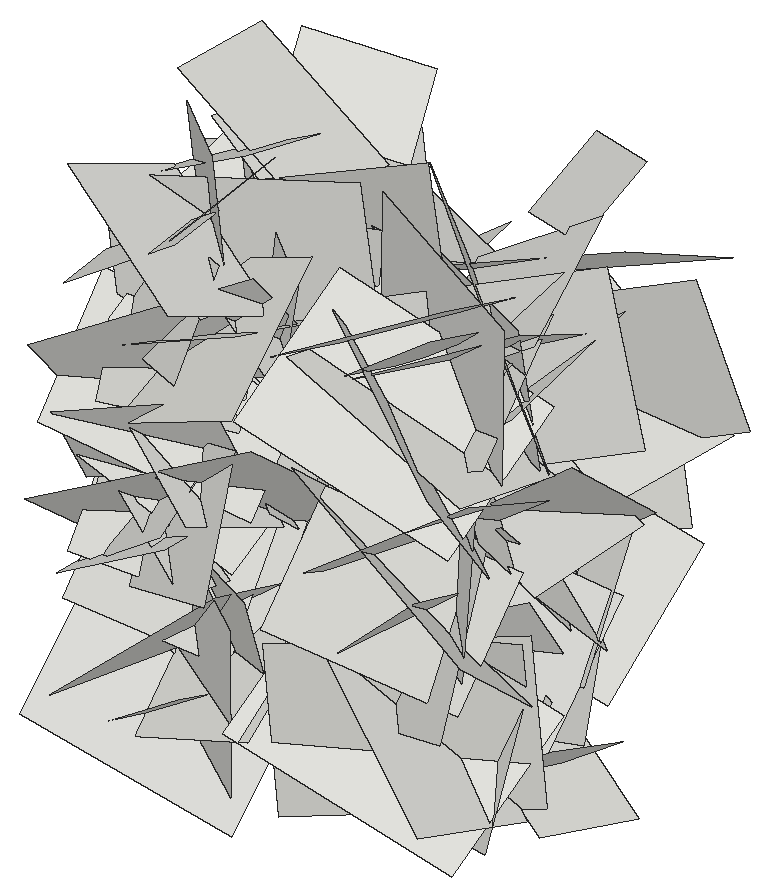
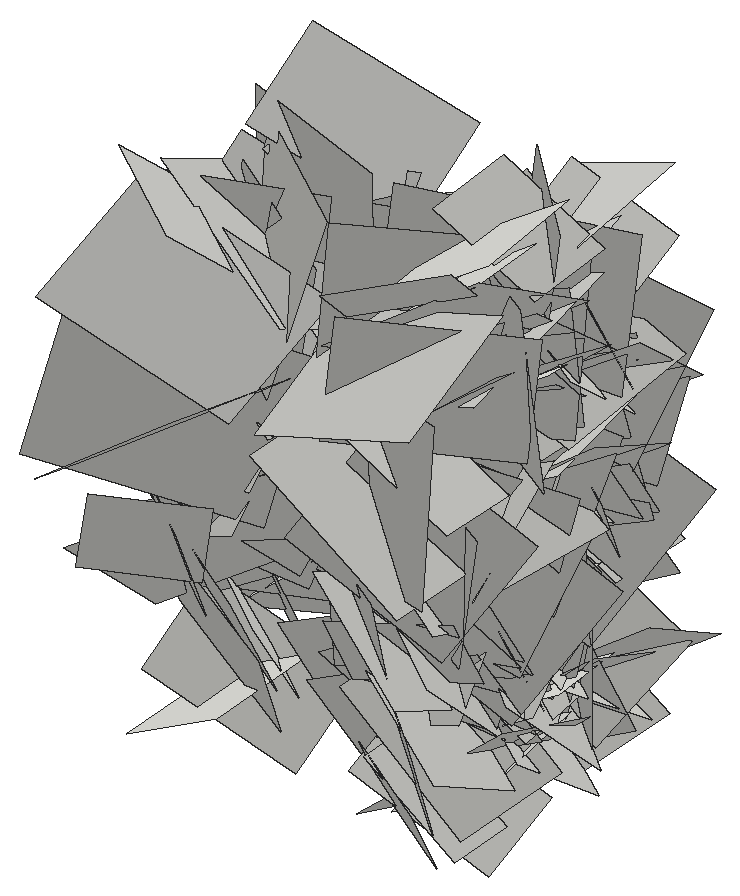
# SketchUp Ruby script. Lengths in inches.
U = 1.inch
M = Sketchup.active_model
def pt(a) = Geom::Point3d.new(a.map { |v| v * U })
def face(e, loops, mat)
  f = e.add_face(loops[0].map { |a| pt(a) })
  loops[1..].each { |l| e.add_face(l.map { |a| pt(a) }).erase! }
  f.material = f.back_material = mat if mat
  f
end
# faces: each face lists its corners as indices into pts; further lists are holes
def faces(e, pts, list, mat = nil) = list.each { |f| face(e, (f[0].is_a?(Array) ? f : [f]).map { |l| l.map { |i| pts[i] } }, mat) }
# xy, xz, yz: faces in a plane at the given z, y or x. An outline is a flat list of corners, or four numbers for a rectangle; further outlines are holes
def ring(l) = l.size == 4 ? [[l[0], l[1]], [l[2], l[1]], [l[2], l[3]], [l[0], l[3]]] : l.each_slice(2).to_a
def flat(e, list, mat, &to3) = list.each { |f| face(e, (f[0].is_a?(Array) ? f : [f]).map { |l| ring(l).map { |u, v| to3.(u, v) } }, mat) }
def xy(e, z, list, mat = nil) = flat(e, list, mat) { |x, y| [x, y, z] }
def xz(e, y, list, mat = nil) = flat(e, list, mat) { |x, z| [x, y, z] }
def yz(e, x, list, mat = nil) = flat(e, list, mat) { |y, z| [x, y, z] }
def lines(e, pts, list) = list.each { |a, b| e.add_line(pt(pts[a]), pt(pts[b])) }
# prism: a flat outline (further loops are holes) pulled along v
def prism(e, loops, v, mat = nil)
  f = face(e, loops, mat); d = Geom::Vector3d.new(v.map { |x| x * U })
  f.pushpull(f.normal.samedirection?(d) ? d.length : -d.length)
end
def box(e, o, s, mat = nil) = prism(e, [[o, [o[0] + s[0], o[1], o[2]], [o[0] + s[0], o[1] + s[1], o[2]], [o[0], o[1] + s[1], o[2]]]], [0, 0, s[2]], mat)
def at(x, y, z, deg = 0) = Geom::Transformation.translation(pt([x, y, z])) * Geom::Transformation.rotation(ORIGIN, Z_AXIS, deg.degrees)
def axes(o, x, y, z) = Geom::Transformation.new([*x, 0, *y, 0, *z, 0, *pt(o).to_a, 1])
def part(name) = M.definitions.add(name)
# library, detail: a bought-in or finely detailed component or shape, given as its bounding box
def library(name, o, s) = part(name).tap { |d| box(d.entities, o, s) }
def detail(e, o, s) = box(e.add_group.entities, o, s)
def put(e, d, t, mat = nil) = e.add_instance(d, t).tap { |i| i.material = mat if mat }
def group(e, t, mat = nil) = e.add_group.tap { |g| g.transformation = t; g.material = mat if mat }.entities
root = M.entities
c1 = part("Component\#6")
p = [[0.01,0,0],[0,3.24,4.54],[4.32,3.24,4.54],[4.33,0,0]]
faces(c1.entities,p,[[0,1,2,3]])
put(root,c1,axes([410.71,139.47,36.72],[0.15825,-0.66033,0.08813],[0.02764,0.09604,0.67542],[0.70562,0.14433,-0.04622]))
put(root,c1,axes([414.68,137.53,34.5],[0.08019,0.3809,0.76753],[-0.04804,0.77121,-0.37826],[-0.90698,-0.00717,0.08789]))
put(root,c1,axes([414.68,137.14,29.31],[-0.00249,0.75761,-0.01469],[-0.08098,-0.01485,-0.75375],[-0.79913,-0.00085,0.07643]))
put(root,c1,axes([414.68,149.44,28.46],[0.01637,-0.35652,-0.61871],[-0.18604,-0.60176,0.34238],[-0.7337,0.14463,-0.10062]))
put(root,c1,axes([410.71,144.76,23.61],[0.10873,-0.7568,0.02149],[-0.01122,0.02025,0.76368],[0.80245,0.10283,0.00777]))
put(root,c1,axes([414.68,139.84,37.375],[-0.13047,0.02824,0.77],[0.11824,0.77221,-0.01049],[-0.80815,0.10842,-0.12584]))
put(root,c1,axes([410.71,147.86,21.63],[-0.08807,-1.00346,0.13322],[-0.11481,0.14172,0.99989],[1.06685,-0.06759,0.1186]))
put(root,c1,axes([410.71,145.6875,25.3],[-0.21495,-0.77208,-0.77151],[-0.06755,-0.77499,0.79232],[1.15499,-0.18901,-0.09724]))
put(root,c1,axes([410.71,141.61,27.46],[-0.15544,0.8369,-0.58263],[-0.03072,-0.5918,-0.84279],[1.08048,0.10358,-0.10778]))
put(root,c1,axes([414.68,146.7,34.04],[0.22474,0.77203,-0.6543],[0.03576,-0.67353,-0.78378],[-1.07212,0.13937,-0.1633]))
put(root,c1,axes([414.68,140.76,35.5625],[-0.0095,0.80566,-0.00603],[0.04784,-0.00552,-0.80445],[-0.85268,-0.00929,-0.04507]))
put(root,c1,axes([414.68,144.98,23.12],[-0.11015,0.70988,0.06167],[0.04855,0.06885,-0.71532],[-0.75374,-0.09931,-0.05509]))
put(root,c1,axes([410.71,147.08,31.53],[-0.0186,0.21399,-0.90436],[-0.04027,-0.90393,-0.21315],[0.98427,-0.03294,-0.02581]))
put(root,c1,axes([410.71,137.85,30.84],[-0.06669,0.91948,0.38333],[-0.06841,0.37952,-0.92095],[1.05374,0.08283,-0.03553]))
put(root,c1,axes([414.68,143.64,28.51],[-0.01569,-0.00258,-0.72773],[-0.02057,-0.72762,0.00297],[-0.77112,0.01947,0.01473]))
put(root,c1,axes([410.71,144.71,33.13],[-0.16995,0.04512,1.05289],[-0.00982,1.0649,-0.04705],[1.11704,0.01623,0.15977]))
put(root,c1,axes([410.71,149.13,24.11],[-0.03147,-0.85153,-0.39996],[-0.02133,-0.3995,0.85202],[0.997,-0.03542,0.00561]))
put(root,c1,axes([410.71,150.98,27.43],[0.11329,-0.77541,-0.3635],[-0.07754,-0.37325,0.77469],[0.90445,0.06513,0.11195]))
put(root,c1,axes([410.71,138.53,29.67],[0.03677,-0.4198,0.69058],[0.10131,0.68849,0.41374],[0.85065,-0.06385,-0.07912]))
put(root,c1,axes([414.68,144.05,31.85],[0.11078,0.17753,-0.74918],[-0.12323,-0.74375,-0.19246],[-0.80677,0.13798,-0.07348]))
put(root,c1,axes([414.68,143.38,25.93],[0.00088,-0.66729,0.07011],[-0.1194,0.06898,0.65784],[-0.70113,-0.01259,-0.11194]))
put(root,c1,axes([414.68,140.84,40.56],[0.05261,0.712,-0.12967],[-0.10362,-0.12219,-0.70833],[-0.7601,0.06594,0.08758]))
put(root,c1,axes([410.71,148.52,32.35],[0.08011,-0.79067,-0.06214],[0.07476,-0.05548,0.79163],[0.83736,0.0806,-0.06473]))
put(root,c1,axes([410.71,142.67,41.25],[-0.05619,0.9574,-0.08237],[0.00834,-0.08206,-0.95886],[1.01856,0.05349,0.00331]))
put(root,c1,axes([414.68,144.6,22.65],[0.17478,-0.82558,-0.09028],[-0.09417,-0.10904,0.83495],[-0.87528,-0.15312,-0.10786]))
put(root,c1,axes([410.71,145.42,24.52],[-0.2647,-0.88765,0.75819],[-0.01358,0.77738,0.90589],[1.23735,-0.18136,0.17214]))
put(root,c1,axes([410.71,141.63,23.18],[-0.01995,1.00092,0.30572],[-0.13829,0.30114,-0.99396],[1.10071,0.05598,-0.11933]))
put(root,c1,axes([414.68,145.6,27.28],[-0.00806,0.29423,-0.56577],[-0.12293,-0.55701,-0.28812],[-0.6647,0.09945,0.06014]))
put(root,c1,axes([410.71,135.48,23.28],[-0.21581,1.04519,0.5846],[-0.09636,0.57779,-1.06467],[1.26577,0.22219,0.01862]))
put(root,c1,axes([414.68,143.53,22.21],[0.15224,-0.84766,-0.36991],[0.10957,-0.35729,0.85887],[-0.97421,-0.17265,0.03879]))
put(root,c1,axes([414.68,137.77,24.11],[0.1419,0.78136,-0.16109],[-0.04598,-0.15597,-0.79258],[-0.84441,0.13979,0.01609]))
put(root,c1,axes([410.71,136.3,32.46],[-0.17238,0.91042,0.71253],[-0.07022,0.71102,-0.92361],[1.22345,0.16908,0.04738]))
put(root,c1,axes([410.71,137.68,27.62],[0.00267,0.49736,0.77514],[0.05686,0.77375,-0.49665],[0.97459,-0.04651,0.02685]))
put(root,c1,axes([410.71,145.12,23.07],[-0.0526,-0.82286,-0.58821],[0.0059,-0.58914,0.82367],[1.07215,-0.03713,-0.03339]))
put(root,c1,axes([414.68,145.7,22.51],[0.08358,0.19729,0.79599],[0.0899,0.79341,-0.20506],[-0.86462,0.10156,0.05562]))
put(root,c1,axes([414.68,146.3,23.53],[0.0913,-0.50535,0.50896],[-0.05568,0.5068,0.51209],[-0.75823,-0.09807,0.02368]))
put(root,c1,axes([414.68,145.72,37.21],[-0.0202,-0.65006,0.07365],[0.02062,0.07308,0.65011],[-0.69316,0.02112,0.01719]))
put(root,c1,axes([414.68,141.16,33.73],[-0.01034,-0.20439,-0.70125],[0.11317,-0.69418,0.20085],[-0.76594,-0.09981,0.03914]))
put(root,c1,axes([410.71,149.17,29.19],[0.22051,-0.77582,-0.34275],[-0.07369,-0.36732,0.78924],[0.89602,0.16072,0.14925]))
put(root,c1,axes([414.68,144.18,33.46],[0.08879,-0.56105,-0.39599],[-0.0694,-0.40364,0.55803],[-0.72461,-0.03009,-0.10197]))
put(root,c1,axes([414.68,136.92,29.78],[-0.03864,0.57092,0.32429],[0.05823,0.3263,-0.56829],[-0.69355,-0.00442,-0.06578]))
put(root,c1,axes([414.68,146.45,21.25],[0.00375,0.2874,0.54008],[-0.0654,0.5375,-0.28562],[-0.64519,-0.05282,0.03209]))
put(root,c1,axes([414.68,144.73,33.27],[0.16555,-0.76551,-0.15352],[-0.02389,-0.16091,0.77946],[-0.82725,-0.14855,-0.05323]))
put(root,c1,axes([410.71,144.65,25.96],[0.15377,0.53431,0.65108],[0.06081,0.65286,-0.54856],[0.89071,-0.13681,-0.07495]))
put(root,c1,axes([414.68,139.71,39.61],[-0.08624,0.67106,-0.00672],[0.16105,0.01183,-0.6586],[-0.69289,-0.08077,-0.15225]))
put(root,c1,axes([410.71,143.41,32.67],[-0.00295,0.89075,-0.72818],[-0.15415,-0.72261,-0.88339],[1.20976,-0.08991,-0.11434]))
put(root,c1,axes([410.71,146.5,19.86],[0.14062,-0.87102,0.18651],[0.03259,0.19294,0.87915],[0.94365,0.12313,-0.05815]))
put(root,c1,axes([410.71,145.05,38.54],[-0.26561,0.06521,-1.32838],[-0.06869,-1.35074,-0.05408],[1.4081,-0.05359,-0.25321]))
put(root,c1,axes([410.71,142.58,23.75],[0.11698,0.88265,-0.34817],[-0.00423,-0.35009,-0.88876],[1.00576,-0.10414,0.03675]))
put(root,c1,axes([410.71,141.41,21.99],[0.04242,-1.10503,0.33762],[-0.18816,0.32793,1.09436],[1.21025,0.08972,0.15831]))
put(root,c1,axes([414.68,145.49,24.46],[0.14807,-0.32942,-0.64401],[-0.00647,-0.65643,0.33444],[-0.76675,-0.05808,-0.12719]))
put(root,c1,axes([410.71,138.75,33.42],[0.07987,0.93748,-0.3836],[-0.04246,-0.3816,-0.94046],[1.07286,-0.0849,-0.00867]))
put(root,c1,axes([414.68,142.8,24.59],[0.06246,-0.31977,0.5346],[-0.03506,0.53462,0.32343],[-0.65938,-0.05871,0.03344]))
put(root,c1,axes([414.68,142.28,27.34],[0.09885,-0.42767,0.49172],[-0.03253,0.4933,0.43487],[-0.69002,-0.08452,0.04994]))
put(root,c1,axes([410.71,139.49,21.74],[0.04906,0.46783,0.90513],[0.0041,0.90598,-0.46846],[1.08001,-0.02469,-0.03934]))
put(root,c1,axes([414.68,149.12,29.1],[0.10824,-0.19319,-0.65872],[0.02698,-0.66445,0.19881],[-0.72715,-0.05341,-0.09068]))
put(root,c1,axes([410.71,145.04,25.97],[-0.0145,-0.85349,0.83598],[-0.13626,0.83223,0.84756],[1.25903,0.08024,0.10136]))
put(root,c1,axes([414.68,141.05,35.76],[0.06877,-0.60814,0.14272],[0.00885,0.14432,0.61116],[-0.66208,-0.06124,0.02299]))
put(root,c1,axes([414.68,149.56,39.6],[0.17317,-0.50739,-0.45031],[-0.03865,-0.46908,0.51531],[-0.71806,-0.09712,-0.13634]))
put(root,c1,axes([414.68,140.39,26.94],[0.03872,-0.62994,0.14227],[0.11345,0.14643,0.62088],[-0.67508,-0.01152,0.1125]))
put(root,c1,axes([414.68,144.97,35.07],[0.07722,-0.5315,-0.34657],[0.05738,-0.34237,0.53643],[-0.67013,-0.09056,0.006]))
put(root,c1,axes([410.71,139.67,30.68],[-0.09112,-0.77438,0.96294],[-0.03313,0.96632,0.77431],[1.3094,-0.02944,0.0866]))
put(root,c1,axes([414.68,147.9,27.03],[0.12769,0.03013,0.63893],[0.01482,0.64988,-0.03329],[-0.67785,0.01989,0.11963]))
put(root,c1,axes([410.71,138.43,27.8],[0.10648,0.28124,1.16655],[-0.16097,1.1642,-0.2676],[1.26174,0.12479,-0.13259]))
put(root,c1,axes([410.71,140.69,35.43],[0.02714,1.22478,0.26938],[-0.1382,0.27058,-1.21783],[1.3221,0.00314,-0.13283]))
put(root,c1,axes([410.71,137.65,40.3125],[0.15365,0.92766,-0.3555],[0.07441,-0.36793,-0.93147],[1.05042,-0.10963,0.11798]))
put(root,c1,axes([410.71,149.09,36.34],[-0.1737,0.35213,-1.24285],[0.08,-1.24806,-0.36356],[1.36694,0.11779,-0.13666]))
put(root,c1,axes([410.71,146.73,29.36],[-0.09029,-1.26195,0.03468],[0.03892,0.03227,1.26436],[1.33761,-0.08612,-0.03444]))
put(root,c1,axes([410.71,141.99,33.2],[0.15631,-0.03731,1.01998],[0.08418,1.02787,0.02612],[1.07863,-0.07482,-0.14985]))
put(root,c1,axes([410.71,141.2,30.22],[0.14348,-0.5033,-0.91823],[0.06175,-0.92081,0.51331],[1.10823,0.11647,0.09028]))
put(root,c1,axes([410.71,143.42,27.33],[0.08667,-0.86973,1.01008],[-0.23887,0.9884,0.86929],[1.39256,0.22367,0.08625]))
put(root,c1,axes([410.71,142.6875,32.73],[-0.11413,-1.14483,0.29443],[0.2702,0.26621,1.12831],[1.22353,-0.16558,-0.2217]))
put(root,c1,axes([410.71,143.97,23.32],[0.18437,0.48358,0.83906],[0.16998,0.82633,-0.50949],[1.01237,-0.22682,-0.06726]))
put(root,c1,axes([410.71,144,25.2],[0.04504,0.58566,0.95802],[0.11757,0.95183,-0.5868],[1.18441,-0.11675,0.02182]))
put(root,c1,axes([410.71,150.86,30.47],[0.14962,-1.13409,-0.09371],[-0.03493,-0.09847,1.14197],[1.20573,0.13788,0.04471]))
put(root,c1,axes([410.71,141.59,27.99],[-0.06396,0.08339,-1.32201],[-0.02487,-1.32324,-0.0824],[1.4039,-0.01964,-0.06169]))
put(root,c1,axes([410.71,145.76,27.48],[0.11303,-0.66031,-0.96553],[-0.02355,-0.9705,0.66125],[1.23968,0.04176,0.1006]))
put(root,c1,axes([410.71,149.48,27.53],[0.05839,-0.93868,-0.8352],[-0.07486,-0.83699,0.93604],[1.32974,-0.0059,0.08937]))
put(root,c1,axes([410.71,141.72,37.36],[0.19445,0.97106,0.50245],[-0.00165,0.50971,-0.98451],[1.15895,-0.1622,-0.0857]))
put(root,c1,axes([410.71,141.71,25.57],[-0.24627,-1.07768,0.84944],[0.21085,0.82598,1.10232],[1.43917,-0.30542,-0.01615]))
put(root,c1,axes([410.71,141.15,27.9],[0.10356,0.25866,-1.08582],[0.18317,-1.08033,-0.24181],[1.16891,0.14638,0.13409]))
put(root,c1,axes([410.71,145.83,38.68],[-0.04371,1.09164,-0.51046],[0.28885,-0.48908,-1.06793],[1.24431,0.15188,0.22998]))
put(root,c1,axes([410.71,140.25,33.3],[-0.10371,-0.10781,1.29757],[0.22808,1.282,0.12274],[1.36119,-0.22303,0.07829]))
put(root,c1,axes([410.71,139.39,34.34],[0.15089,0.92592,0.71699],[0.08883,0.71236,-0.93659],[1.23815,-0.16395,-0.02018]))
put(root,c1,axes([410.71,142.42,32.89],[0.18672,-0.42722,1.28431],[-0.1337,1.28432,0.44452],[1.42847,0.17605,-0.12627]))
put(root,c1,axes([410.71,142.63,35.02],[0.11092,-0.98462,-0.77371],[0.1183,-0.76598,0.98988],[1.32209,0.15114,-0.02366]))
put(root,c1,axes([410.71,137.42,26.21],[0.14568,0.69276,1.17725],[0.03045,1.18146,-0.69859],[1.44759,-0.09457,-0.10377]))
put(root,c1,axes([410.71,143.09,24.72],[0.05768,-1.1082,-0.74759],[0.23067,-0.73089,1.09928],[1.3981,0.16631,-0.15052]))
put(root,c1,axes([410.71,141,38.04],[0.14868,1.2474,-0.57055],[0.09146,-0.58042,-1.24775],[1.45112,-0.09122,0.1371]))
put(root,c1,axes([424.49,141,38.04],[-0.14868,1.2474,-0.57055],[-0.09146,-0.58042,-1.24775],[-1.45112,-0.09122,0.1371]))
put(root,c1,axes([424.49,143.09,24.72],[-0.05768,-1.1082,-0.74759],[-0.23067,-0.73089,1.09928],[-1.3981,0.16631,-0.15052]))
put(root,c1,axes([424.49,137.42,26.21],[-0.14568,0.69276,1.17725],[-0.03045,1.18146,-0.69859],[-1.44759,-0.09457,-0.10377]))
put(root,c1,axes([424.49,142.63,35.02],[-0.11092,-0.98462,-0.77371],[-0.1183,-0.76598,0.98988],[-1.32209,0.15114,-0.02366]))
put(root,c1,axes([424.49,142.42,32.89],[-0.18672,-0.42722,1.28431],[0.1337,1.28432,0.44452],[-1.42847,0.17605,-0.12627]))
put(root,c1,axes([424.49,139.39,34.34],[-0.15089,0.92592,0.71699],[-0.08883,0.71236,-0.93659],[-1.23815,-0.16395,-0.02018]))
put(root,c1,axes([424.49,140.25,33.3],[0.10371,-0.10781,1.29757],[-0.22808,1.282,0.12274],[-1.36119,-0.22303,0.07829]))
put(root,c1,axes([424.49,145.83,38.68],[0.04371,1.09164,-0.51046],[-0.28885,-0.48908,-1.06793],[-1.24431,0.15188,0.22998]))
put(root,c1,axes([424.49,141.15,27.9],[-0.10356,0.25866,-1.08582],[-0.18317,-1.08033,-0.24181],[-1.16891,0.14638,0.13409]))
put(root,c1,axes([424.49,141.71,25.57],[0.24627,-1.07768,0.84944],[-0.21085,0.82598,1.10232],[-1.43917,-0.30542,-0.01615]))
put(root,c1,axes([424.49,141.72,37.36],[-0.19445,0.97106,0.50245],[0.00165,0.50971,-0.98451],[-1.15895,-0.1622,-0.0857]))
put(root,c1,axes([424.49,149.48,27.53],[-0.05839,-0.93868,-0.8352],[0.07486,-0.83699,0.93604],[-1.32974,-0.0059,0.08937]))
put(root,c1,axes([424.49,145.76,27.48],[-0.11303,-0.66031,-0.96553],[0.02355,-0.9705,0.66125],[-1.23968,0.04176,0.1006]))
put(root,c1,axes([424.49,141.59,27.99],[0.06396,0.08339,-1.32201],[0.02487,-1.32324,-0.0824],[-1.4039,-0.01964,-0.06169]))
put(root,c1,axes([424.49,150.86,30.47],[-0.14962,-1.13409,-0.09371],[0.03493,-0.09847,1.14197],[-1.20573,0.13788,0.04471]))
put(root,c1,axes([424.49,144,25.2],[-0.04504,0.58566,0.95802],[-0.11757,0.95183,-0.5868],[-1.18441,-0.11675,0.02182]))
put(root,c1,axes([424.49,143.97,23.32],[-0.18437,0.48358,0.83906],[-0.16998,0.82633,-0.50949],[-1.01237,-0.22682,-0.06726]))
put(root,c1,axes([424.49,142.6875,32.73],[0.11413,-1.14483,0.29443],[-0.2702,0.26621,1.12831],[-1.22353,-0.16558,-0.2217]))
put(root,c1,axes([424.49,143.42,27.33],[-0.08667,-0.86973,1.01008],[0.23887,0.9884,0.86929],[-1.39256,0.22367,0.08625]))
put(root,c1,axes([424.49,141.2,30.22],[-0.14348,-0.5033,-0.91823],[-0.06175,-0.92081,0.51331],[-1.10823,0.11647,0.09028]))
put(root,c1,axes([424.49,141.99,33.2],[-0.15631,-0.03731,1.01998],[-0.08418,1.02787,0.02612],[-1.07863,-0.07482,-0.14985]))
put(root,c1,axes([424.49,146.73,29.36],[0.09029,-1.26195,0.03468],[-0.03892,0.03227,1.26436],[-1.33761,-0.08612,-0.03444]))
put(root,c1,axes([424.49,149.09,36.34],[0.1737,0.35213,-1.24285],[-0.08,-1.24806,-0.36356],[-1.36694,0.11779,-0.13666]))
put(root,c1,axes([424.49,137.65,40.3125],[-0.15365,0.92766,-0.3555],[-0.07441,-0.36793,-0.93147],[-1.05042,-0.10963,0.11798]))
put(root,c1,axes([424.49,140.69,35.43],[-0.02714,1.22478,0.26938],[0.1382,0.27058,-1.21783],[-1.3221,0.00314,-0.13283]))
put(root,c1,axes([424.49,138.43,27.8],[-0.10648,0.28124,1.16655],[0.16097,1.1642,-0.2676],[-1.26174,0.12479,-0.13259]))
put(root,c1,axes([420.52,147.9,27.03],[-0.12769,0.03013,0.63893],[-0.01482,0.64988,-0.03329],[0.67785,0.01989,0.11963]))
put(root,c1,axes([424.49,139.67,30.68],[0.09112,-0.77438,0.96294],[0.03313,0.96632,0.77431],[-1.3094,-0.02944,0.0866]))
put(root,c1,axes([420.52,144.97,35.07],[-0.07722,-0.5315,-0.34657],[-0.05738,-0.34237,0.53643],[0.67013,-0.09056,0.006]))
put(root,c1,axes([420.52,140.39,26.94],[-0.03872,-0.62994,0.14227],[-0.11345,0.14643,0.62088],[0.67508,-0.01152,0.1125]))
put(root,c1,axes([420.52,149.56,39.6],[-0.17317,-0.50739,-0.45031],[0.03865,-0.46908,0.51531],[0.71806,-0.09712,-0.13634]))
put(root,c1,axes([420.52,141.05,35.76],[-0.06877,-0.60814,0.14272],[-0.00885,0.14432,0.61116],[0.66208,-0.06124,0.02299]))
put(root,c1,axes([424.49,145.04,25.97],[0.0145,-0.85349,0.83598],[0.13626,0.83223,0.84756],[-1.25903,0.08024,0.10136]))
put(root,c1,axes([420.52,149.12,29.1],[-0.10824,-0.19319,-0.65872],[-0.02698,-0.66445,0.19881],[0.72715,-0.05341,-0.09068]))
put(root,c1,axes([424.49,139.49,21.74],[-0.04906,0.46783,0.90513],[-0.0041,0.90598,-0.46846],[-1.08001,-0.02469,-0.03934]))
put(root,c1,axes([420.52,142.28,27.34],[-0.09885,-0.42767,0.49172],[0.03253,0.4933,0.43487],[0.69002,-0.08452,0.04994]))
put(root,c1,axes([420.52,142.8,24.59],[-0.06246,-0.31977,0.5346],[0.03506,0.53462,0.32343],[0.65938,-0.05871,0.03344]))
put(root,c1,axes([424.49,138.75,33.42],[-0.07987,0.93748,-0.3836],[0.04246,-0.3816,-0.94046],[-1.07286,-0.0849,-0.00867]))
put(root,c1,axes([420.52,145.49,24.46],[-0.14807,-0.32942,-0.64401],[0.00647,-0.65643,0.33444],[0.76675,-0.05808,-0.12719]))
put(root,c1,axes([424.49,141.41,21.99],[-0.04242,-1.10503,0.33762],[0.18816,0.32793,1.09436],[-1.21025,0.08972,0.15831]))
put(root,c1,axes([424.49,142.58,23.75],[-0.11698,0.88265,-0.34817],[0.00423,-0.35009,-0.88876],[-1.00576,-0.10414,0.03675]))
put(root,c1,axes([424.49,145.05,38.54],[0.26561,0.06521,-1.32838],[0.06869,-1.35074,-0.05408],[-1.4081,-0.05359,-0.25321]))
put(root,c1,axes([424.49,146.5,19.86],[-0.14062,-0.87102,0.18651],[-0.03259,0.19294,0.87915],[-0.94365,0.12313,-0.05815]))
put(root,c1,axes([424.49,143.41,32.67],[0.00295,0.89075,-0.72818],[0.15415,-0.72261,-0.88339],[-1.20976,-0.08991,-0.11434]))
